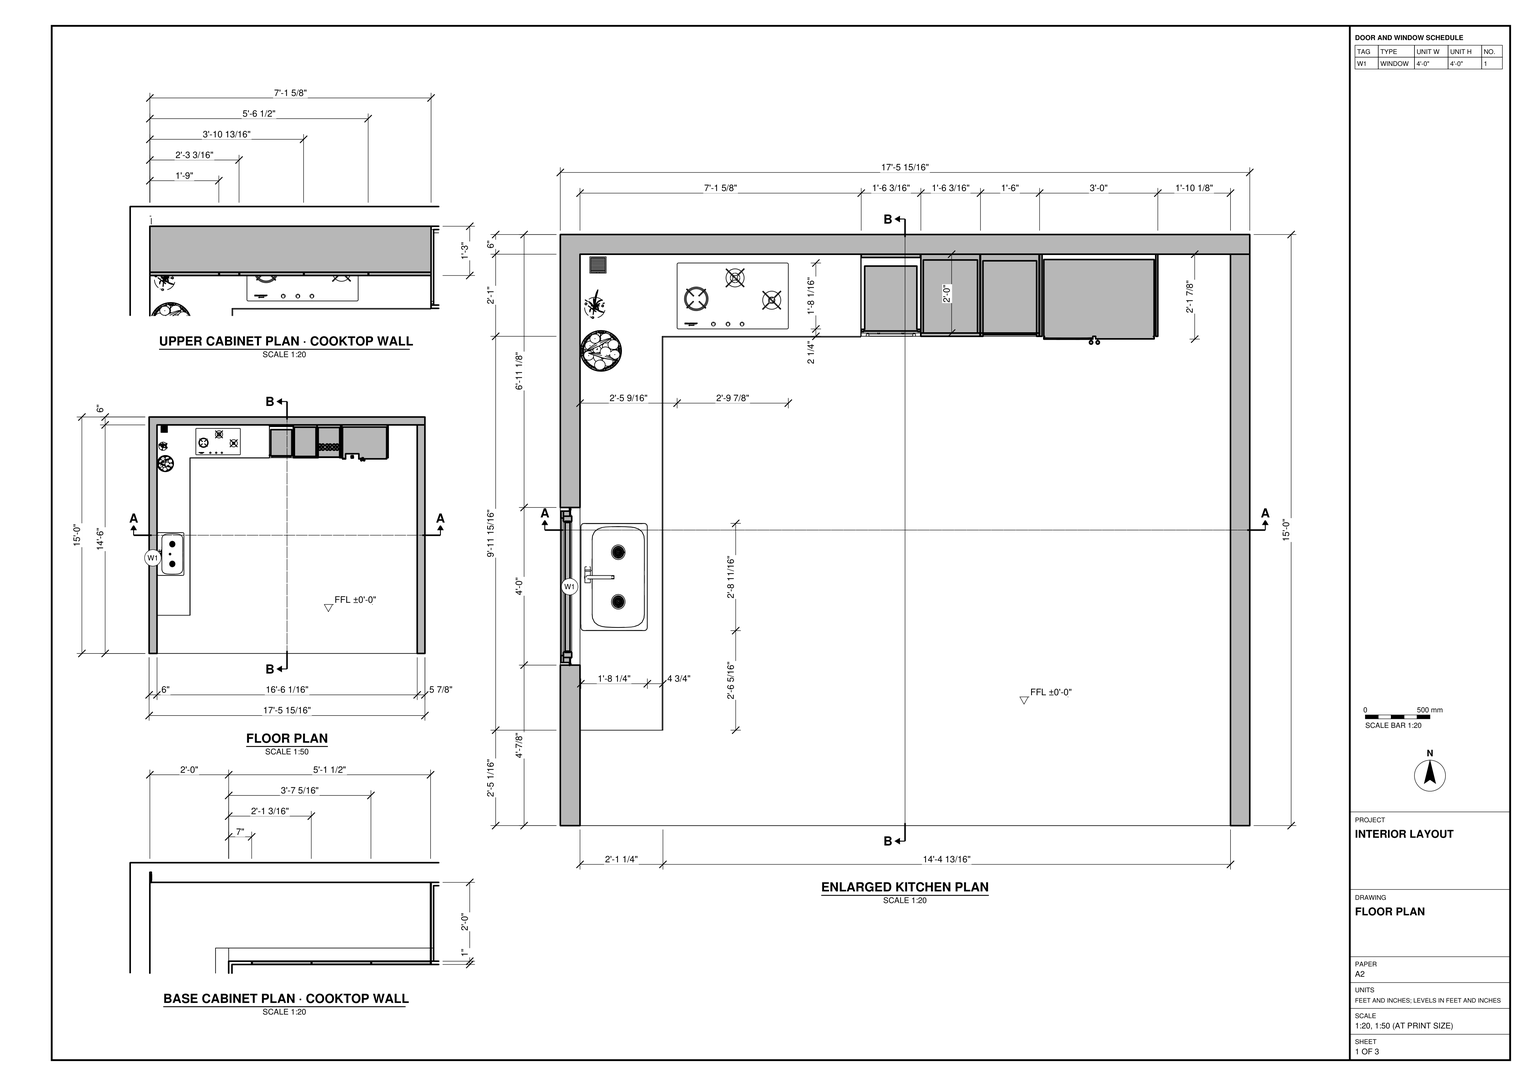
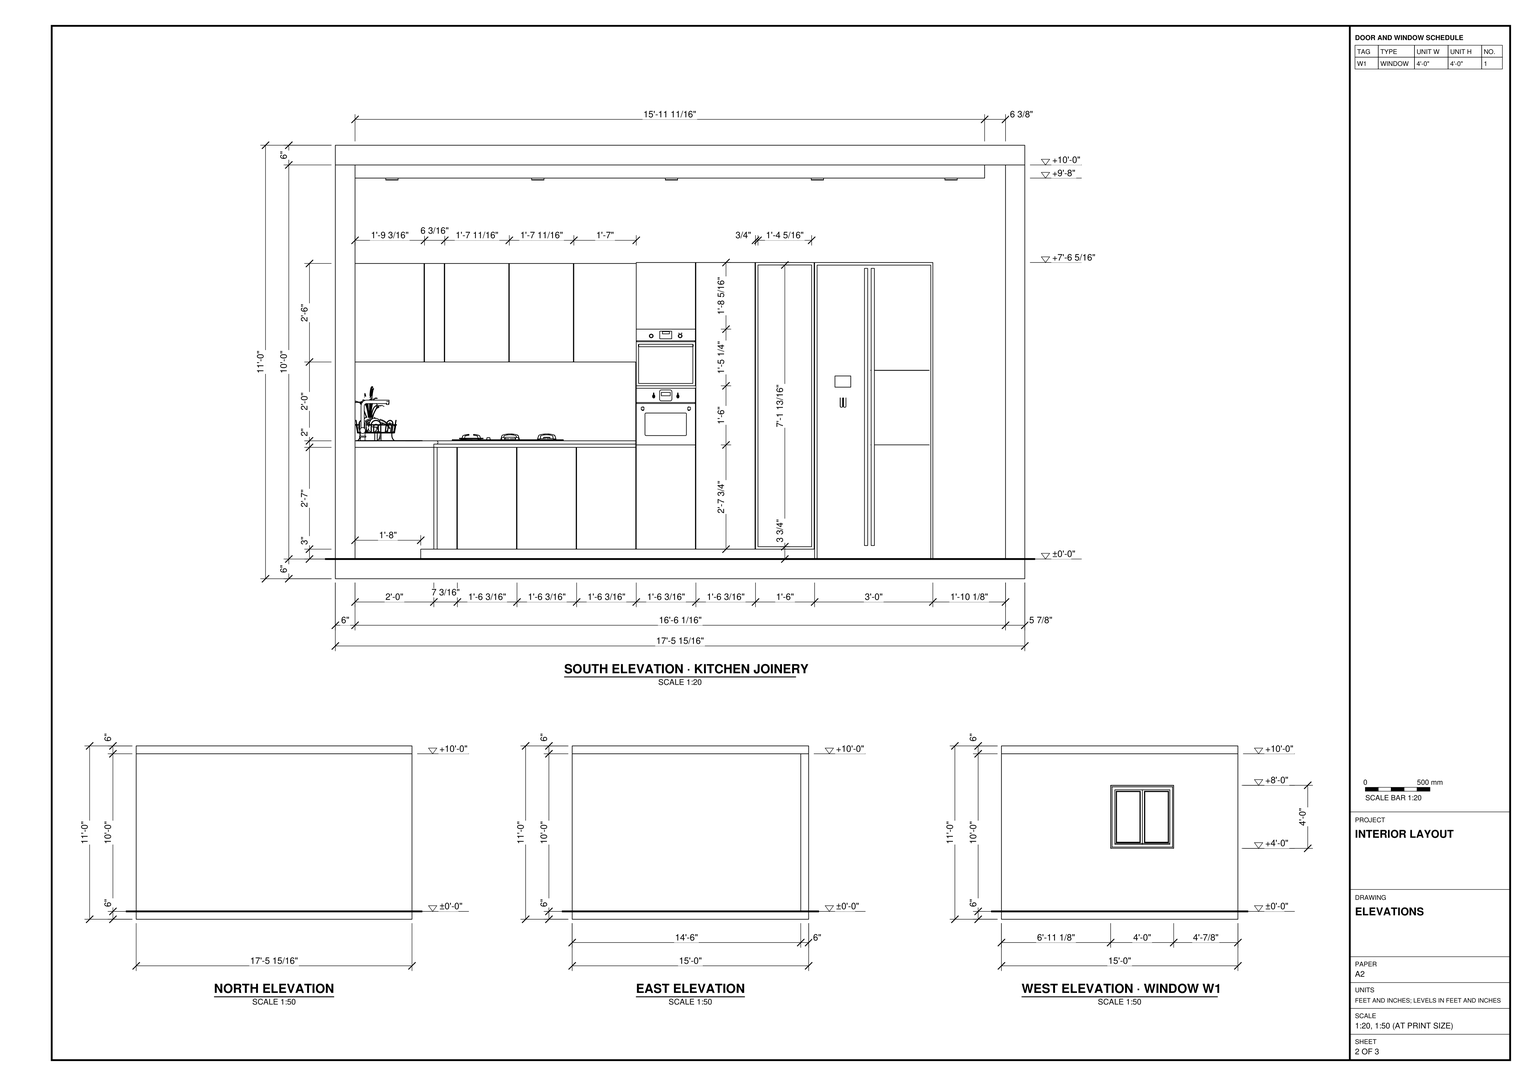
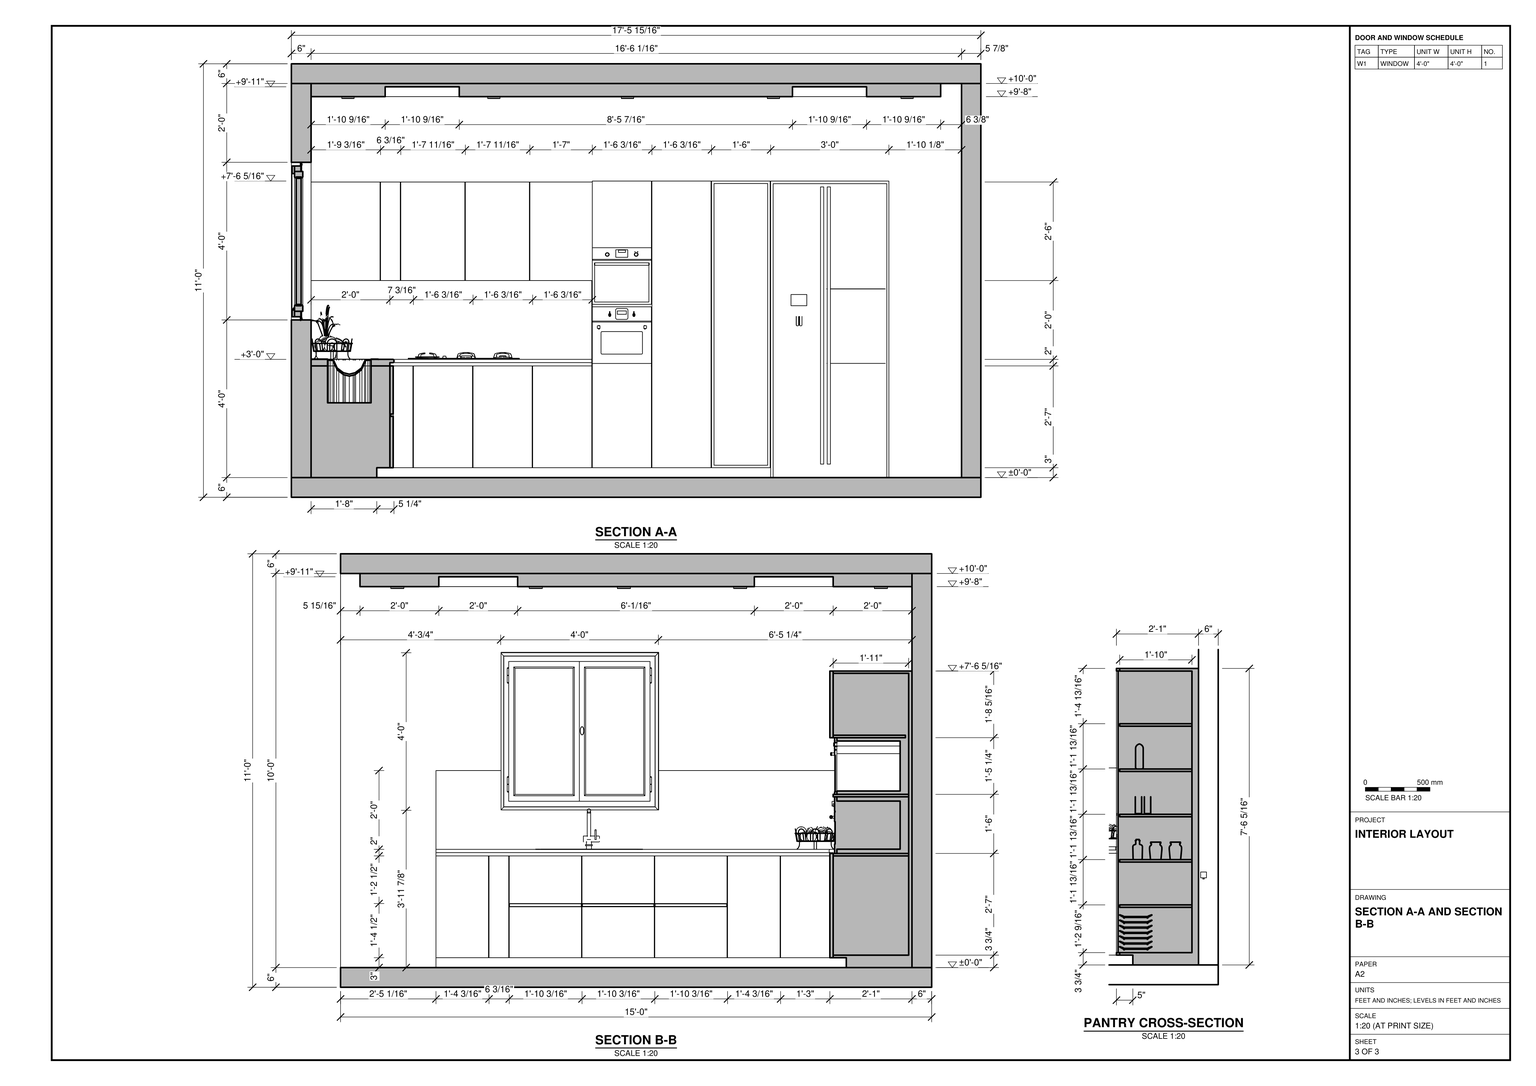
Build the kitchen in SketchUp from task_files/diagram_01.pdf. Work in feet and inches. The room shell measures 17'-5 15/16" across the cooktop wall, 15'-0" from back to front and 11'-0" high overall. Set the finished floor at ±0'-0". Model the back and side walls at the thicknesses drawn, leaving the front open as shown in plan. Include the floor slab, overhead slab and stepped ceiling underside shown in section.

Use the enlarged plan to lay out the L-shaped worktop. Fit the sink and faucet into the return beneath the west window, and place the cooktop on the adjoining run. Use the cabinet plans for the upper and base cabinet depths, and the elevations and sections for the cabinet fronts, drawers, recessed plinths and worktop height. Continue the cooktop wall with the stacked appliance cabinet, tall storage and refrigerator, leaving the gap shown at the end. Model the pantry shelves from the cross-section. Appliances, decor and loose countertop items may be any suitable library components placed where shown.

Keep the shell elements and each joinery or furniture piece in separate groups or components, and use components for repeated parts. Save one SketchUp model as output_files/l_shaped_kitchen_with_a_window_and_pantry.skp.

# SketchUp Ruby script. Lengths in inches.
U = 1.inch
M = Sketchup.active_model
def pt(a) = Geom::Point3d.new(a.map { |v| v * U })
def face(e, loops, mat)
  f = e.add_face(loops[0].map { |a| pt(a) })
  loops[1..].each { |l| e.add_face(l.map { |a| pt(a) }).erase! }
  f.material = f.back_material = mat if mat
  f
end
# faces: each face lists its corners as indices into pts; further lists are holes
def faces(e, pts, list, mat = nil) = list.each { |f| face(e, (f[0].is_a?(Array) ? f : [f]).map { |l| l.map { |i| pts[i] } }, mat) }
# xy, xz, yz: faces in a plane at the given z, y or x. An outline is a flat list of corners, or four numbers for a rectangle; further outlines are holes
def ring(l) = l.size == 4 ? [[l[0], l[1]], [l[2], l[1]], [l[2], l[3]], [l[0], l[3]]] : l.each_slice(2).to_a
def flat(e, list, mat, &to3) = list.each { |f| face(e, (f[0].is_a?(Array) ? f : [f]).map { |l| ring(l).map { |u, v| to3.(u, v) } }, mat) }
def xy(e, z, list, mat = nil) = flat(e, list, mat) { |x, y| [x, y, z] }
def xz(e, y, list, mat = nil) = flat(e, list, mat) { |x, z| [x, y, z] }
def yz(e, x, list, mat = nil) = flat(e, list, mat) { |y, z| [x, y, z] }
def lines(e, pts, list) = list.each { |a, b| e.add_line(pt(pts[a]), pt(pts[b])) }
# prism: a flat outline (further loops are holes) pulled along v
def prism(e, loops, v, mat = nil)
  f = face(e, loops, mat); d = Geom::Vector3d.new(v.map { |x| x * U })
  f.pushpull(f.normal.samedirection?(d) ? d.length : -d.length)
end
def box(e, o, s, mat = nil) = prism(e, [[o, [o[0] + s[0], o[1], o[2]], [o[0] + s[0], o[1] + s[1], o[2]], [o[0], o[1] + s[1], o[2]]]], [0, 0, s[2]], mat)
def at(x, y, z, deg = 0) = Geom::Transformation.translation(pt([x, y, z])) * Geom::Transformation.rotation(ORIGIN, Z_AXIS, deg.degrees)
def axes(o, x, y, z) = Geom::Transformation.new([*x, 0, *y, 0, *z, 0, *pt(o).to_a, 1])
def part(name) = M.definitions.add(name)
# library, detail: a bought-in or finely detailed component or shape, given as its bounding box
def library(name, o, s) = part(name).tap { |d| box(d.entities, o, s) }
def detail(e, o, s) = box(e.add_group.entities, o, s)
def put(e, d, t, mat = nil) = e.add_instance(d, t).tap { |i| i.material = mat if mat }
def group(e, t, mat = nil) = e.add_group.tap { |g| g.transformation = t; g.material = mat if mat }.entities
root = M.entities
M.materials.add("Generic1").color = [196, 159, 159]
M.materials.add("Glass (Bening)").color = [254, 254, 254]
M.materials.add("[0057_DarkKhaki]").color = [189, 183, 107]
M.materials.add("[0079_Teal]").color = [0, 128, 128]
M.materials.add("[0123_DarkMagenta]").color = [132, 0, 132]
M.materials.add("[0136_Charcoal]").color = [173, 71, 127]
M.materials.add("[Carrera Marble]").color = [207, 207, 207]
M.materials.add("[Color D01]").color = [209, 195, 182]
M.materials.add("[Color D02]1").color = [145, 138, 121]
M.materials.add("[Color M04]").color = [142, 142, 142]
M.materials.add("[Field Square Tile]").color = [217, 201, 169]
M.materials.add("[Ornate Tile 02]").color = [198, 198, 198]
M.materials.add("[Translucent Glass Gray]").color = [128, 128, 128]
M.materials.add("[Wood Veneer 01]").color = [120, 70, 37]
M.materials.add("cupboard upper").color = [255, 255, 255]
M.materials.add("wood cork").color = [180, 131, 85]
c1 = part("Cabinet shelf")
box(c1.entities,[0,0,0],[16.34,22,0.75])
c2 = library("3-MICRO H40 CLC2",[0,-1.47,0],[23.5,21.86,15.63])
c3 = library("5-FOUR H60 CLC2",[0,-1.15,0],[23.5,21.54,23.5])
c4 = library("RF006",[-8.76,-6.5,0],[17.54,12.67,35.43])
c5 = library("Double bowl sink",[-0.47,-0.25,-9.95],[20.24,32.66,22.28])
c6 = library("window",[-69.79,-2.12,-0.98],[49.21,5.34,45.27])
c7 = library("7-TABLE DE CUISSON CLC2",[-16.93,-10.04,0.13],[33.86,20.08,1.97])
c8 = library("7-VASEFLEURS CLC2",[-5.69,-5.69,0],[10.79,12.36,17.9])
c9 = library("3-PNGFRUITS CLC2",[-6.29,-6.27,0],[12.57,12.48,7.4])
c10 = library("4-PRISEELC CLC2",[-1.57,-1.58,0],[3.14,3.14,0.51])
c11 = library("Group\#5",[0,4.54,0],[175.94,144.95,90.29])
c12 = part("coaster3")
prism(c12.entities,[[[2.67,0.2,1.33],[2.62,0.2,0.99],[2.49,0.2,0.67],[2.28,0.2,0.39],[2,0.2,0.18],[1.68,0.2,0.05],[1.33,0.2,0],[0.99,0.2,0.05],[0.67,0.2,0.18],[0.39,0.2,0.39],[0.18,0.2,0.67],[0.05,0.2,0.99],[0,0.2,1.33],[0.05,0.2,1.68],[0.18,0.2,2],[0.39,0.2,2.28],[0.67,0.2,2.49],[0.99,0.2,2.62],[1.33,0.2,2.67],[1.68,0.2,2.62],[2,0.2,2.49],[2.28,0.2,2.28],[2.49,0.2,2],[2.62,0.2,1.68]]],[0,-0.2,0])
c13 = part("Long Drink glas")
xy(c13.entities,0.08,[[5.85,0,5.6,0.03,5.36,0.13,5.16,0.29,5,0.49,4.9,0.73,4.87,0.98,4.9,1.24,5,1.48,5.16,1.68,5.36,1.84,5.6,1.93,5.85,1.97,6.11,1.93,6.34,1.84,6.55,1.68,6.7,1.48,6.8,1.24,6.84,0.98,6.8,0.73,6.7,0.49,6.55,0.29,6.34,0.13,6.11,0.03]])
xy(c13.entities,0.27,[[5.89,0.02,6.14,0.0625,6.36,0.17,6.56,0.33,6.7,0.54,6.79,0.77,6.8125,1.02,6.81,1.05,6.77,1.27,6.67,1.5,6.51,1.69,6.3,1.84,6.0625,1.92,5.8125,1.95,5.57,1.9,5.34,1.8,5.14,1.64,5,1.43,4.91,1.2,4.89,0.95,4.9,0.86,4.93,0.7,5.04,0.47,5.2,0.28,5.4,0.13,5.64,0.04]])
xy(c13.entities,5.39,[[[5.85,0,6.11,0.03,6.34,0.13,6.55,0.29,6.7,0.49,6.8,0.73,6.84,0.98,6.83,1.05,6.82,1.11,6.8,1.24,6.7,1.48,6.55,1.68,6.34,1.84,6.11,1.93,5.85,1.97,5.6,1.93,5.36,1.84,5.16,1.68,5,1.48,4.9,1.24,4.87,0.98,4.88,0.86,4.9,0.73,5,0.49,5.16,0.29,5.36,0.13,5.6,0.03],[5.89,0.02,5.64,0.04,5.4,0.13,5.2,0.28,5.04,0.47,4.93,0.7,4.9,0.86,4.89,0.95,4.91,1.2,5,1.43,5.14,1.64,5.34,1.8,5.57,1.9,5.8125,1.95,6.0625,1.92,6.3,1.84,6.51,1.69,6.67,1.5,6.77,1.27,6.81,1.05,6.8125,1.02,6.79,0.77,6.7,0.54,6.56,0.33,6.36,0.17,6.14,0.0625]]])
p = [[5.36,0.13,0.08],[5.6,0.03,0.08],[5.6,0.03,5.39],[5.36,0.13,5.39],[5.85,0,0.08],[5.85,0,5.39],
  [6.11,0.03,0.08],[6.11,0.03,5.39],[6.34,0.13,0.08],[6.34,0.13,5.39],[5.16,0.29,0.08],[5.16,0.29,5.39],
  [6.55,0.29,0.08],[6.55,0.29,5.39],[5,0.49,0.08],[5,0.49,5.39],[6.7,0.49,0.08],[6.7,0.49,5.39],
  [4.9,0.73,0.08],[4.95,0.61,5.39],[4.9,0.73,5.39],[6.8,0.73,0.08],[6.8,0.73,5.39],[4.87,0.98,0.08],
  [4.88,0.86,5.39],[4.87,0.98,5.39],[6.84,0.98,0.08],[6.84,0.98,5.39],[4.9,1.24,0.08],[4.9,1.24,5.39],
  [6.8,1.24,0.08],[6.8,1.24,5.39],[6.82,1.11,5.39],[6.83,1.05,5.39],[5,1.48,0.08],[5,1.48,5.39],
  [6.7,1.48,0.08],[6.7,1.48,5.39],[5.16,1.68,0.08],[5.16,1.68,5.39],[6.55,1.68,0.08],[6.55,1.68,5.39],
  [5.36,1.84,0.08],[5.36,1.84,5.39],[6.34,1.84,0.08],[6.34,1.84,5.39],[5.6,1.93,0.08],[5.6,1.93,5.39],
  [6.11,1.93,0.08],[6.11,1.93,5.39],[5.85,1.97,0.08],[5.85,1.97,5.39],[5.64,0.04,0.27],[5.4,0.13,0.27],
  [5.4,0.13,5.39],[5.64,0.04,5.39],[5.89,0.02,0.27],[5.89,0.02,5.39],[6.14,0.0625,0.27],[6.14,0.0625,5.39],
  [5.2,0.28,0.27],[5.2,0.28,5.39],[6.36,0.17,0.27],[6.36,0.17,5.39],[6.56,0.33,0.27],[6.56,0.33,5.39],
  [5.04,0.47,0.27],[5.04,0.47,5.39],[6.7,0.54,0.27],[6.7,0.54,5.39],[4.93,0.7,0.27],[4.93,0.7,5.39],
  [6.79,0.77,0.27],[6.79,0.77,5.39],[4.9,0.86,0.27],[4.9,0.86,5.39],[6.8125,1.02,0.27],[6.8125,1.02,5.39],
  [4.89,0.95,0.27],[4.89,0.95,5.39],[4.91,1.2,0.27],[4.91,1.2,5.39],[6.81,1.05,0.27],[6.81,1.05,5.39],
  [6.77,1.27,0.27],[6.77,1.27,5.39],[5,1.43,0.27],[5,1.43,5.39],[6.67,1.5,0.27],[6.67,1.5,5.39],
  [5.14,1.64,0.27],[5.14,1.64,5.39],[6.51,1.69,0.27],[6.51,1.69,5.39],[5.34,1.8,0.27],[5.34,1.8,5.39],
  [6.3,1.84,0.27],[6.3,1.84,5.39],[5.57,1.9,0.27],[5.57,1.9,5.39],[6.0625,1.92,0.27],[6.0625,1.92,5.39],
  [5.8125,1.95,0.27],[5.8125,1.95,5.39]]
faces(c13.entities,p,[[0,1,2,3],[1,4,5,2],[4,6,7,5],[6,8,9,7],[10,0,3,11],[8,12,13,9],[14,10,11,15],[12,16,17,13],
  [18,14,15,19,20],[16,21,22,17],[23,18,20,24,25],[21,26,27,22],[28,23,25,29],[26,30,31,32,33,27],[34,28,29,35],[30,36,37,31],
  [38,34,35,39],[36,40,41,37],[42,38,39,43],[40,44,45,41],[46,42,43,47],[44,48,49,45],[50,46,47,51],[48,50,51,49],
  [52,53,54,55],[56,52,55,57],[58,56,57,59],[53,60,61,54],[62,58,59,63],[64,62,63,65],[60,66,67,61],[68,64,65,69],
  [66,70,71,67],[72,68,69,73],[70,74,75,71],[76,72,73,77],[74,78,79,75],[78,80,81,79],[82,76,77,83],[84,82,83,85],
  [80,86,87,81],[88,84,85,89],[86,90,91,87],[92,88,89,93],[90,94,95,91],[96,92,93,97],[94,98,99,95],[100,96,97,101],
  [98,102,103,99],[102,100,101,103]])
c14 = part("Group\#286")
put(c14.entities,c13,at(0,9.59,-0.08,-90),"Glass (Bening)")
put(c14.entities,c13,at(0,6.84,-0.08,-90),"Glass (Bening)")
put(c14.entities,c13,at(2.41,9.59,-0.08,-90),"Glass (Bening)")
put(c14.entities,c13,at(2.41,6.84,-0.08,-90),"Glass (Bening)")
c15 = library("Group\#304",[0,0,0],[9.84,9.84,10.67])
c16 = library("Group\#307",[-0.58,-0.58,0],[9.39,13.47,7.89])
c17 = library("Group\#19",[0,0,0],[15.26,7.83,11.77])
c18 = library("Group\#20",[0,0,0],[13.61,3.47,11.45])
c19 = library("Group\#21",[0,0,0],[14.7,14.86,6.14])
c20 = library("Recessed light",[-0.01,-0.01,0],[4,4,0.6])
xy(root,34,[[[6,29.06,6,174,91.47,174,91.47,150,30,150,30,29.06],[17.64,60.32,18.8,60.34,19.2,60.35,19.57,60.36,20.83,60.42,21.49,60.46,22.26,60.58,22.63,60.64,23.29,60.87,23.8125,61.05,24.56,61.64,24.875,61.89,25.29,62.77,25.48,63.17,25.62,64.43,25.62,86.97,25.48,88.23,25.29,88.64,24.875,89.51,24.56,89.76,23.8125,90.35,23.29,90.53,22.63,90.77,22.26,90.82,21.49,90.94,20.83,90.98,19.57,91.04,19.2,91.04,18.8,91.06,17.64,91.08,16.47,91.06,16.08,91.04,15.71,91.04,14.44,90.98,13.78,90.94,13.01,90.82,12.64,90.77,11.98,90.53,11.46,90.35,10.72,89.76,10.4,89.51,9.98,88.64,9.79,88.23,9.67,86.97,9.67,64.43,9.79,63.17,9.98,62.77,10.4,61.89,10.72,61.64,11.46,61.05,11.98,60.87,12.64,60.64,13.01,60.58,13.78,60.46,14.44,60.42,15.71,60.36,16.08,60.35,16.47,60.34]]],"[Carrera Marble]")
xy(root,35,[[30,29.06,31,149],[30,149,91.47,150]],"[Carrera Marble]")
xy(root,36,[[[6,29.06,31,29.06,31,149,91.47,149,91.47,174,6,174],[17.64,60.32,16.47,60.34,16.08,60.35,15.71,60.36,14.44,60.42,13.78,60.46,13.01,60.58,12.64,60.64,11.98,60.87,11.46,61.05,10.72,61.64,10.4,61.89,9.98,62.77,9.79,63.17,9.67,64.43,9.67,86.97,9.79,88.23,9.98,88.64,10.4,89.51,10.72,89.76,11.46,90.35,11.98,90.53,12.64,90.77,13.01,90.82,13.78,90.94,14.44,90.98,15.71,91.04,16.08,91.04,16.47,91.06,17.64,91.08,18.8,91.06,19.2,91.04,19.57,91.04,20.83,90.98,21.49,90.94,22.26,90.82,22.63,90.77,23.29,90.53,23.8125,90.35,24.56,89.76,24.875,89.51,25.29,88.64,25.48,88.23,25.62,86.97,25.62,64.43,25.48,63.17,25.29,62.77,24.875,61.89,24.56,61.64,23.8125,61.05,23.29,60.87,22.63,60.64,22.26,60.58,21.49,60.46,20.83,60.42,19.57,60.36,19.2,60.35,18.8,60.34],[8.32,74.86,8.13,74.89,7.96,74.96,7.8125,75.09,7.7,75.25,7.625,75.43,7.6,75.63,7.625,75.83,7.7,76.02,7.8125,76.18,7.96,76.3,8.13,76.38,8.32,76.41,8.51,76.38,8.68,76.3,8.83,76.18,8.94,76.02,9.01,75.83,9.04,75.63,9.01,75.43,8.94,75.25,8.83,75.09,8.68,74.96,8.51,74.89]],[8.32,74.86,8.51,74.89,8.68,74.96,8.83,75.09,8.94,75.25,9.01,75.43,9.04,75.63,9.01,75.83,8.94,76.02,8.83,76.18,8.68,76.3,8.51,76.38,8.32,76.41,8.13,76.38,7.96,76.3,7.8125,76.18,7.7,76.02,7.625,75.83,7.6,75.63,7.625,75.43,7.7,75.25,7.8125,75.09,7.96,74.96,8.13,74.89]],"[Carrera Marble]")
xz(root,29.06,[[6,34,30,34,30,35,31,35,31,36,6,36],[31,35,31.07,35.0625,31.13,35.14,31.18,35.22,31.22,35.31,31.24,35.4,31.25,35.5,31.24,35.6,31.22,35.69,31.18,35.78,31.13,35.86,31.07,35.9375,31,36]],"[Carrera Marble]")
xz(root,70.13,[[25.62,34,25.62,34,25.62,36,25.62,36]],"[Carrera Marble]")
xz(root,78.71,[[9.67,34,9.67,34,9.67,36,9.67,36]],"[Carrera Marble]")
xz(root,81.27,[[9.67,34,9.67,34,9.67,36,9.67,36]],"[Carrera Marble]")
xz(root,91.04,[[15.71,34,16.08,36],[19.2,34,19.57,36]],"[Carrera Marble]")
xz(root,150,[[30,34,91.47,35]],"[Carrera Marble]")
xz(root,174,[[6,34,91.47,36]],"[Carrera Marble]")
yz(root,6,[[29.06,34,174,36]],"[Carrera Marble]")
yz(root,9.67,[[64.43,34,70.13,36],[70.13,34,72.13,36],[72.13,34,73.8,36],[73.8,34,75.17,36],[75.17,34,76.23,36],
  [76.23,34,77.6,36],[77.6,34,78.71,36],[78.71,34,81.27,36],[81.27,34,86.97,36]],"[Carrera Marble]")
yz(root,25.62,[[64.43,34,70.13,36],[70.13,34,72.6875,36],[72.6875,34,72.69,36],[72.69,34,73.8,36],[73.8,34,75.17,36],
  [75.17,34,76.23,36],[76.23,34,77.6,36],[77.6,34,79.27,36],[79.27,34,81.27,36],[81.27,34,86.97,36]],"[Carrera Marble]")
yz(root,30,[[29.06,34,150,35]],"[Carrera Marble]")
yz(root,91.47,[[150,34,174,34,174,36,149,36,148.93,35.9375,148.87,35.86,148.82,35.78,148.78,35.69,148.76,35.6,148.75,35.5,148.76,35.4,148.78,35.31,148.82,35.22,148.87,35.14,148.93,35.0625,149,35,150,35]],"[Carrera Marble]")
# 165 loose lines left out
p = [[15.71,60.36,36],[16.08,60.35,36],[16.08,60.35,34],[15.71,60.36,34],[16.47,60.34,36],[16.47,60.34,34],
  [17.64,60.32,36],[17.64,60.32,34],[18.8,60.34,36],[18.8,60.34,34],[19.2,60.35,36],[19.2,60.35,34],
  [19.57,60.36,36],[19.57,60.36,34],[13.78,60.46,36],[14.44,60.42,36],[14.44,60.42,34],[13.78,60.46,34],
  [20.83,60.42,36],[20.83,60.42,34],[21.49,60.46,36],[21.49,60.46,34],[13.01,60.58,36],[13.01,60.58,34],
  [22.26,60.58,36],[22.26,60.58,34],[11.98,60.87,36],[12.64,60.64,36],[12.64,60.64,34],[11.98,60.87,34],
  [22.63,60.64,36],[22.63,60.64,34],[23.29,60.87,36],[23.29,60.87,34],[11.46,61.05,36],[11.46,61.05,34],
  [23.8125,61.05,36],[23.8125,61.05,34],[10.72,61.64,36],[10.72,61.64,34],[24.56,61.64,36],[24.56,61.64,34],
  [10.4,61.89,36],[10.4,61.89,34],[24.875,61.89,36],[24.875,61.89,34],[9.98,62.77,36],[9.98,62.77,34],
  [25.29,62.77,36],[25.29,62.77,34],[9.79,63.17,36],[9.79,63.17,34],[25.48,63.17,36],[25.48,63.17,34],
  [9.67,64.43,36],[9.67,64.43,34],[25.58,64.07,36],[25.58,64.07,34],[25.62,64.43,36],[25.62,64.43,34],
  [9.79,88.23,36],[9.67,86.97,36],[9.67,86.97,34],[9.79,88.23,34],[25.62,86.97,36],[25.58,87.33,36],
  [25.58,87.33,34],[25.62,86.97,34],[25.48,88.23,36],[25.48,88.23,34],[9.98,88.64,36],[9.98,88.64,34],
  [25.29,88.64,36],[25.29,88.64,34],[10.4,89.51,36],[10.4,89.51,34],[24.875,89.51,36],[24.875,89.51,34],
  [10.72,89.76,36],[10.72,89.76,34],[24.56,89.76,36],[24.56,89.76,34],[11.46,90.35,36],[11.46,90.35,34],
  [23.8125,90.35,36],[23.8125,90.35,34],[11.98,90.53,36],[11.98,90.53,34],[23.29,90.53,36],[23.29,90.53,34],
  [12.64,90.77,36],[12.64,90.77,34],[22.63,90.77,36],[22.63,90.77,34],[13.01,90.82,36],[13.01,90.82,34],
  [13.78,90.94,36],[13.78,90.94,34],[22.26,90.82,36],[21.49,90.94,36],[21.49,90.94,34],[22.26,90.82,34],
  [14.44,90.98,36],[14.44,90.98,34],[20.83,90.98,36],[20.83,90.98,34],[15.71,91.04,36],[15.71,91.04,34],
  [16.47,91.06,36],[16.08,91.04,36],[16.08,91.04,34],[16.47,91.06,34],[19.2,91.04,36],[18.8,91.06,36],
  [18.8,91.06,34],[19.2,91.04,34],[19.57,91.04,36],[19.57,91.04,34],[17.64,91.08,36],[17.64,91.08,34],
  [31.07,29.06,35.0625],[31,29.06,35],[31,149,35],[31.07,148.93,35.0625],[91.47,149,35],[91.47,148.93,35.0625],
  [31.13,29.06,35.14],[31.13,148.87,35.14],[31.18,29.06,35.22],[31.18,148.82,35.22],[91.47,148.87,35.14],[91.47,148.82,35.22],
  [31.22,29.06,35.31],[31.22,148.78,35.31],[91.47,148.78,35.31],[31.24,29.06,35.4],[31.24,148.76,35.4],[91.47,148.76,35.4],
  [31.25,29.06,35.5],[31.25,148.75,35.5],[91.47,148.75,35.5],[31.24,29.06,35.6],[31.24,148.76,35.6],[91.47,148.76,35.6],
  [31.22,29.06,35.69],[31.22,148.78,35.69],[91.47,148.78,35.69],[31.18,29.06,35.78],[31.18,148.82,35.78],[91.47,148.82,35.78],
  [31.13,29.06,35.86],[31.13,148.87,35.86],[91.47,148.87,35.86],[31,29.06,36],[31.07,29.06,35.9375],[31.07,148.93,35.9375],
  [31,149,36],[91.47,148.93,35.9375],[91.47,149,36]]
faces(root,p,[[0,1,2,3],[1,4,5,2],[4,6,7,5],[6,8,9,7],[8,10,11,9],[10,12,13,11],[14,15,16,17],[15,0,3,16],
  [12,18,19,13],[18,20,21,19],[22,14,17,23],[20,24,25,21],[26,27,28,29],[27,22,23,28],[24,30,31,25],[30,32,33,31],
  [34,26,29,35],[32,36,37,33],[38,34,35,39],[36,40,41,37],[42,38,39,43],[40,44,45,41],[46,42,43,47],[44,48,49,45],
  [50,46,47,51],[48,52,53,49],[54,50,51,55],[52,56,57,53],[56,58,59,57],[60,61,62,63],[64,65,66,67],[65,68,69,66],
  [70,60,63,71],[68,72,73,69],[74,70,71,75],[72,76,77,73],[78,74,75,79],[76,80,81,77],[82,78,79,83],[80,84,85,81],
  [86,82,83,87],[84,88,89,85],[90,86,87,91],[88,92,93,89],[94,90,91,95],[96,94,95,97],[98,99,100,101],[92,98,101,93],
  [102,96,97,103],[99,104,105,100],[106,102,103,107],[108,109,110,111],[112,113,114,115],[104,116,117,105],[118,108,111,119],[113,118,119,114],
  [120,121,122,123],[123,122,124,125],[126,120,123,127],[128,126,127,129],[129,127,130,131],[127,123,125,130],[132,128,129,133],[133,129,131,134],
  [135,132,133,136],[136,133,134,137],[138,135,136,139],[139,136,137,140],[141,138,139,142],[142,139,140,143],[144,141,142,145],[145,142,143,146],
  [147,144,145,148],[148,145,146,149],[150,147,148,151],[151,148,149,152],[153,154,155,156],[154,150,151,155],[156,155,157,158],[155,151,152,157]],"[Carrera Marble]")
put(root,c1,at(128.69,150,17.54))
put(root,c1,at(128.69,150,31.33))
put(root,c1,at(128.69,150,45.125))
put(root,c1,at(128.69,150,58.92))
put(root,c1,at(128.69,150,72.71))
put(root,c2,axes([91.63,150.4375,34.75],[0.76583,0,0],[0,0.97847,0],[0,0,1.10365]))
put(root,c3,axes([91.63,150.4375,52.75],[0.76583,0,0],[0,0.97847,0],[0,0,0.73392]))
put(root,c4,axes([164.03,159.83,0],[1.91729,0,0],[0,2.03386,0],[0,0,2.51178]))
put(root,c5,axes([26.03,91.79,36.04],[-1,0,0],[0,-1,0.00108],[0,0.00108,1]))
put(root,c6,axes([3.4,116.85,48.92],[0,0.97564,0],[-0.99,0,0],[0,0,1.06007]))
put(root,c7,at(52.5,161.29,36))
put(root,c8,at(10.52,157.68,36))
put(root,c9,at(12.39,144.6,36))
put(root,c10,axes([6,175.53,27.43],[0,1,0],[0,0,1],[1,0,0]))
g1 = group(root,at(0,0,-6),"Generic1")
xy(g1,0,[[0,0,209.94,180]])
xy(g1,6,[[0,0,209.94,180]],"[Field Square Tile]")
xz(g1,0,[[0,0,209.94,6]])
xz(g1,180,[[0,0,209.94,6]])
yz(g1,0,[[0,0,180,6]])
yz(g1,209.94,[[0,0,180,6]])
put(root,c11,at(6,24.51,0),"[Field Square Tile]")
g2 = group(root,at(91.63,149,3),"[Color D02]1")
box(g2,[0,0,0],[18,1,31.75])
g3 = group(root,at(92.4,150,70))
box(g3,[0,0,0],[16.45,22,0.75])
g4 = group(root,at(91.63,149,57),"[Color D02]1")
box(g4,[0,0,13],[18,1,20.29])
g5 = group(root,at(91.63,150,34))
g6 = group(g5,at(0.77,0,0))
box(g6,[-0.77,0,0],[18.15,23,0.75])
g7 = group(g5,at(0.77,0,18))
box(g7,[-0.77,0,0],[18.15,23,0.75])
g8 = group(root,at(6,160,60))
box(g8,[0,0,0],[85.63,14,30],"[Color D01]")
g9 = group(root,at(6,159,60),"[Color D01]")
box(g9,[46.97,0,0],[19.5,1,30],"[Color D01]")
xy(g9,0,[[0,0,21,1],[21.16,0,27.16,1],[27.31,0,46.81,1]])
xy(g9,0,[[66.63,0,85.63,1]],"cupboard upper")
xy(g9,30,[[0,0,21,1],[21.16,0,27.16,1],[27.31,0,46.81,1]])
xy(g9,30,[[66.63,0,85.63,1]],"[Color D01]")
xz(g9,0,[[0,0,21,30],[21.16,0,27.16,30],[27.31,0,46.81,30],[66.63,0,85.63,30]],"[Color D01]")
xz(g9,1,[[0,0,21,30],[21.16,0,27.16,30],[27.31,0,46.81,30]])
xz(g9,1,[[66.63,0,85.63,30]],"cupboard upper")
yz(g9,0,[[0,0,1,30]])
yz(g9,21,[[0,0,1,30]])
yz(g9,21.16,[[0,0,1,30]])
yz(g9,27.16,[[0,0,1,30]])
yz(g9,27.31,[[0,0,1,30]])
yz(g9,46.81,[[0,0,1,30]])
yz(g9,66.63,[[0,0,1,30]],"cupboard upper")
yz(g9,85.63,[[0,0,1,30]],"cupboard upper")
g10 = group(root,at(30,24.51,3),"[Color D02]1")
prism(g10,[[[0,125.49,0],[7,125.49,0],[7,124.49,0],[1,124.49,0],[1,109.49,0],[0,109.49,0]]],[0,0,31])
box(g10,[0,93.33,0],[1,16,31])
box(g10,[0,20.7,0],[1,6,31])
box(g10,[0,4.54,0],[1,16,31])
box(g10,[43.47,124.49,0],[18,1,31])
box(g10,[25.31,124.49,0],[18,1,31])
box(g10,[7.16,124.49,0],[18,1,31])
xy(g10,0,[[0,26.86,1,48.86],[0,49.02,1,71.02],[0,71.17,1,93.17]])
xy(g10,15.6,[[0.25,26.96,1,48.76]],"[0136_Charcoal]")
xy(g10,15.625,[[0.25,71.3,1,93.05]],"[0136_Charcoal]")
xy(g10,15.65,[[0.25,49.17,1,70.86]],"[0136_Charcoal]")
xy(g10,16.35,[[0.25,49.17,1,70.86]],"[0136_Charcoal]")
xy(g10,16.375,[[0.25,71.3,1,93.05]],"[0136_Charcoal]")
xy(g10,16.4,[[0.25,26.96,1,48.76]],"[0136_Charcoal]")
xy(g10,31,[[0,26.86,1,48.86],[0,49.02,1,71.02],[0,71.17,1,93.17]])
xz(g10,26.86,[[0,0,1,31]])
xz(g10,26.96,[[0.25,15.6,1,16.4]],"[0136_Charcoal]")
xz(g10,48.76,[[0.25,15.6,1,16.4]],"[0136_Charcoal]")
xz(g10,48.86,[[0,0,1,31]])
xz(g10,49.02,[[0,0,1,31]])
xz(g10,49.17,[[0.25,15.65,1,16.35]],"[0136_Charcoal]")
xz(g10,70.86,[[0.25,15.65,1,16.35]],"[0136_Charcoal]")
xz(g10,71.02,[[0,0,1,31]])
xz(g10,71.17,[[0,0,1,31]])
xz(g10,71.3,[[0.25,15.625,1,16.375]],"[0136_Charcoal]")
xz(g10,93.05,[[0.25,15.625,1,16.375]],"[0136_Charcoal]")
xz(g10,93.17,[[0,0,1,31]])
yz(g10,0,[[26.86,0,48.86,31],[49.02,0,71.02,31],[71.17,0,93.17,31]])
yz(g10,0.25,[[26.96,15.6,48.76,16.4],[71.3,15.625,93.05,16.375],[49.17,15.65,70.86,16.35]],"[0136_Charcoal]")
yz(g10,1,[[26.86,0,48.86,15.5],[49.02,0,71.02,15.5],[71.17,0,93.17,15.5],[[26.86,15.5,48.86,16.5],[26.96,15.6,48.76,16.4]],[[49.02,15.5,71.02,16.5],[49.17,15.65,70.86,16.35]],
  [[71.17,15.5,93.17,16.5],[71.3,15.625,93.05,16.375]],[26.86,16.5,48.86,31],[49.02,16.5,71.02,31],[71.17,16.5,93.17,31]])
g11 = group(root,at(127.94,149,3))
g12 = group(g11,at(0,1,0),"[Color M04]")
g13 = group(g12,at(0,-1,0))
prism(g13,[[[17.84,1,87.29],[17.84,1,0],[0,1,0],[0,1,87.29]],[[17.09,1,0.75],[17.09,1,86.54],[0.75,1,86.54],[0.75,1,0.75]]],[0,-1,0],"[0123_DarkMagenta]")
g14 = group(g11,at(0.75,0.5,0.75))
xz(g14,0,[[0,0,16.34,85.79]],"[Translucent Glass Gray]")
g15 = group(root,at(8.99,168.25,36))
put(g15,c12,axes([0.3,0.28,0.53],[1.64,0,0],[0,1.64,0],[0,0,1.64]),"wood cork")
put(g15,c12,axes([0.3,0.63,0.53],[1.64,0,0],[0,1.64,0],[0,0,1.64]),"wood cork")
put(g15,c12,axes([0.3,0.99,0.53],[1.64,0,0],[0,1.64,0],[0,0,1.64]),"wood cork")
put(g15,c12,axes([0.3,1.34,0.53],[1.64,0,0],[0,1.64,0],[0,0,1.64]),"wood cork")
put(g15,c12,axes([0.3,2.41,0.53],[1.64,0,0],[0,1.64,0],[0,0,1.64]),"wood cork")
put(g15,c12,axes([0.3,1.7,0.53],[1.64,0,0],[0,1.64,0],[0,0,1.64]),"wood cork")
put(g15,c12,axes([0.3,2.05,0.53],[1.64,0,0],[0,1.64,0],[0,0,1.64]),"wood cork")
put(g15,c12,axes([0.3,2.76,0.53],[1.64,0,0],[0,1.64,0],[0,0,1.64]),"wood cork")
put(g15,c12,axes([0.3,3.12,0.53],[1.64,0,0],[0,1.64,0],[0,0,1.64]),"wood cork")
put(g15,c12,axes([0.3,3.47,0.53],[1.64,0,0],[0,1.64,0],[0,0,1.64]),"wood cork")
put(g15,c12,axes([0.3,3.83,0.53],[1.64,0,0],[0,1.64,0],[0,0,1.64]),"wood cork")
put(g15,c12,axes([0.3,4.18,0.53],[1.64,0,0],[0,1.64,0],[0,0,1.64]),"wood cork")
g16 = group(g15,at(0,0,0),"[Wood Veneer 01]")
xy(g16,0,[[0,0,4.97,4.97]])
xy(g16,0.45,[[0.3,0.25,4.67,0.7]])
xy(g16,2.71,[[0,0,2.03,0,2.03,0.25,0.3,0.25,0.3,4.67,4.67,4.67,4.67,0.25,2.9375,0.25,2.9375,0,4.97,0,4.97,4.97,0,4.97]])
xz(g16,0,[[0,0,4.97,0,4.97,2.71,2.9375,2.71,2.9375,1.36,2.92,1.24,2.88,1.13,2.81,1.04,2.71,0.96,2.6,0.92,2.49,0.9,2.37,0.92,2.26,0.96,2.17,1.04,2.09,1.13,2.05,1.24,2.03,1.36,2.03,2.71,0,2.71]])
xz(g16,0.25,[[0.3,0.45,0.3,2.71,2.03,2.71,2.03,1.36,2.05,1.24,2.09,1.13,2.17,1.04,2.26,0.96,2.37,0.92,2.49,0.9,2.49,0.45],[2.49,0.45,2.49,0.9,2.6,0.92,2.71,0.96,2.81,1.04,2.88,1.13,2.92,1.24,2.9375,1.36,2.9375,2.71,4.67,2.71,4.67,0.45]])
xz(g16,4.97,[[0,0,4.97,2.71]])
yz(g16,0,[[0,0,4.97,2.71]])
yz(g16,0.3,[[0.25,0.45,0.7,2.71]])
yz(g16,2.03,[[0,1.36,0.25,2.71]])
yz(g16,2.9375,[[0,1.36,0.25,2.71]])
yz(g16,4.67,[[0.25,0.45,0.7,2.71]])
yz(g16,4.97,[[0,0,4.97,2.71]])
p = [[2.26,0,0.96],[2.37,0,0.92],[2.37,0.25,0.92],[2.26,0.25,0.96],[2.49,0,0.9],[2.49,0.25,0.9],
  [2.6,0,0.92],[2.6,0.25,0.92],[2.71,0,0.96],[2.71,0.25,0.96],[2.09,0,1.13],[2.17,0,1.04],
  [2.17,0.25,1.04],[2.09,0.25,1.13],[2.81,0,1.04],[2.81,0.25,1.04],[2.88,0,1.13],[2.88,0.25,1.13],
  [2.05,0,1.24],[2.05,0.25,1.24],[2.92,0,1.24],[2.92,0.25,1.24],[2.03,0,1.36],[2.03,0.25,1.36],
  [2.9375,0,1.36],[2.9375,0.25,1.36]]
faces(g16,p,[[0,1,2,3],[1,4,5,2],[4,6,7,5],[6,8,9,7],[10,11,12,13],[11,0,3,12],[8,14,15,9],[14,16,17,15],
  [18,10,13,19],[16,20,21,17],[22,18,19,23],[20,24,25,21]])
g17 = group(root,at(128.94,154.74,45.9))
put(g17,c14,at(0,0,0))
put(g17,c14,at(5.5,0,0))
put(g17,c14,at(10.8125,0,0))
g18 = group(root,at(0,0,0),"[Ornate Tile 02]")
xy(g18,0,[[0,0,0,180,209.94,180,209.94,174,6,174,6,0]])
xy(g18,48,[[0,48.875,6,96.875]],"Generic1")
xy(g18,96,[[0,48.875,6,96.875]],"Generic1")
xy(g18,120,[[0,0,6,0,6,174,209.94,174,209.94,180,0,180]],"Generic1")
xz(g18,0,[[0,0,6,120]],"Generic1")
xz(g18,48.875,[[0,48,6,96]],"Generic1")
xz(g18,96.875,[[0,48,6,96]],"Generic1")
xz(g18,174,[[6,36,91.47,60]])
xz(g18,174,[[6,0,209.94,0,209.94,120,6,120,6,60,91.47,60,91.47,36,6,36]],"Generic1")
xz(g18,180,[[0,0,209.94,120]],"Generic1")
yz(g18,0,[[[0,0,180,120],[48.875,48,96.875,96]]],"Generic1")
yz(g18,6,[[29.06,36,174,36,174,60,96.875,60,96.875,48,48.875,48,48.875,60,29.06,60]])
yz(g18,6,[[0,0,174,0,174,36,29.06,36,29.06,60,48.875,60,48.875,96,96.875,96,96.875,60,174,60,174,120,0,120]],"Generic1")
yz(g18,209.94,[[174,0,180,120]],"Generic1")
put(root,c15,at(130.35,149.97,4.6))
put(root,c16,at(131.48,152.53,18.625))
put(root,c17,at(128.69,152.32,73.46))
put(root,c18,at(129.96,154.26,59.67))
put(root,c19,at(129.99,153.98,32.08))
g19 = group(root,at(109.79,149,3),"[Color D02]1")
box(g19,[0,0,0],[18,1,87.29])
g20 = group(root,at(0,0,120),"Generic1")
box(g20,[0,0,0],[209.94,180,6])
g21 = group(root,at(6,5.92,116),"[0057_DarkKhaki]")
xy(g21,0,[[[0,0,191.71,168.08],[22.56,24,169.15,144.08]],[45.12,48,146.59,120.08]],"[0057_DarkKhaki]")
xy(g21,3,[[[22.56,24,169.15,144.08],[45.12,48,146.59,120.08]]],"[0079_Teal]")
xy(g21,4,[[0,0,191.71,168.08]],"[0057_DarkKhaki]")
xz(g21,0,[[0,0,191.71,4]],"[0057_DarkKhaki]")
xz(g21,24,[[22.56,0,169.15,3]],"[0057_DarkKhaki]")
xz(g21,48,[[45.12,0,146.59,3]],"[0057_DarkKhaki]")
xz(g21,120.08,[[45.12,0,146.59,3]],"[0057_DarkKhaki]")
xz(g21,144.08,[[22.56,0,169.15,3]],"[0057_DarkKhaki]")
xz(g21,168.08,[[0,0,191.71,4]],"[0057_DarkKhaki]")
yz(g21,0,[[0,0,168.08,4]],"[0057_DarkKhaki]")
yz(g21,22.56,[[24,0,144.08,3]],"[0057_DarkKhaki]")
yz(g21,45.12,[[48,0,120.08,3]],"[0057_DarkKhaki]")
yz(g21,146.59,[[48,0,120.08,3]],"[0057_DarkKhaki]")
yz(g21,169.15,[[24,0,144.08,3]],"[0057_DarkKhaki]")
yz(g21,191.71,[[0,0,168.08,4]],"[0057_DarkKhaki]")
put(g21,c20,axes([142.66,51.53,0],[-0.94,0,0],[0,1,0],[0,0,-1]))
put(g21,c20,axes([142.66,113.78,0],[-0.94,0,0],[0,1,0],[0,0,-1]))
put(g21,c20,axes([57.53,51.53,0],[-0.94,0,0],[0,1,0],[0,0,-1]))
put(g21,c20,axes([57.53,113.78,0],[-0.94,0,0],[0,1,0],[0,0,-1]))
put(g21,c20,axes([183.36,78.37,0],[-0.94,0,0],[0,1,0],[0,0,-1]))
put(g21,c20,axes([183.36,9.38,0],[-0.94,0,0],[0,1,0],[0,0,-1]))
put(g21,c20,axes([183.36,156.63,0],[-0.94,0,0],[0,1,0],[0,0,-1]))
put(g21,c20,axes([98.23,156.63,0],[-0.94,0,0],[0,1,0],[0,0,-1]))
put(g21,c20,axes([98.23,9.38,0],[-0.94,0,0],[0,1,0],[0,0,-1]))
put(g21,c20,axes([13.1,156.63,0],[-0.94,0,0],[0,1,0],[0,0,-1]))
put(g21,c20,axes([13.1,9.38,0],[-0.94,0,0],[0,1,0],[0,0,-1]))
put(g21,c20,axes([13.1,78.37,0],[-0.94,0,0],[0,1,0],[0,0,-1]))
g22 = group(root,at(204.07,0,0),"Generic1")
box(g22,[0,0,0],[5.875,174,120])
